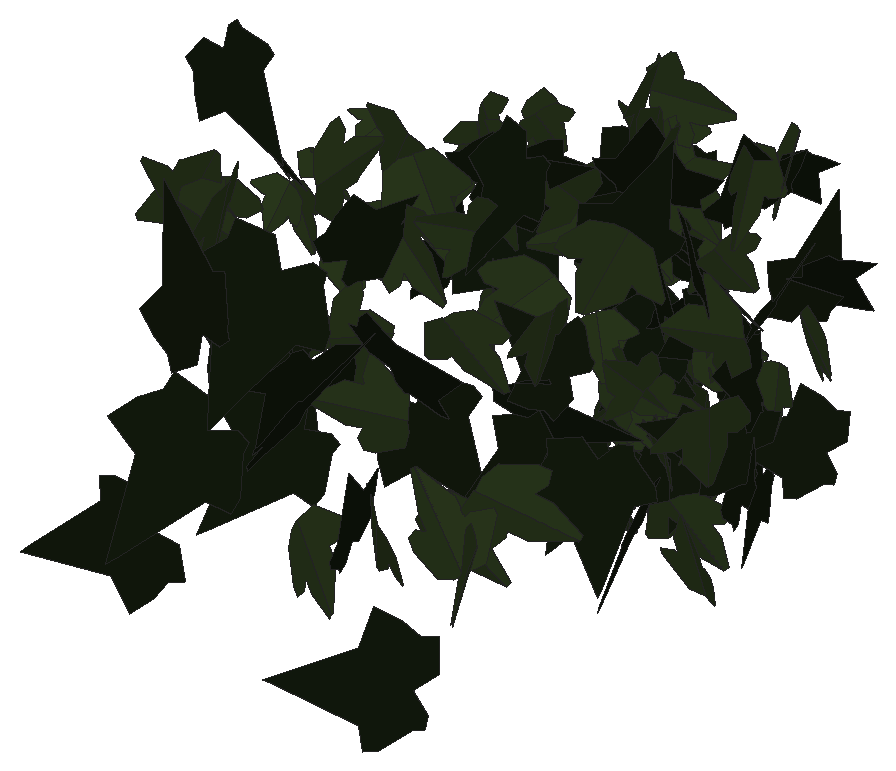
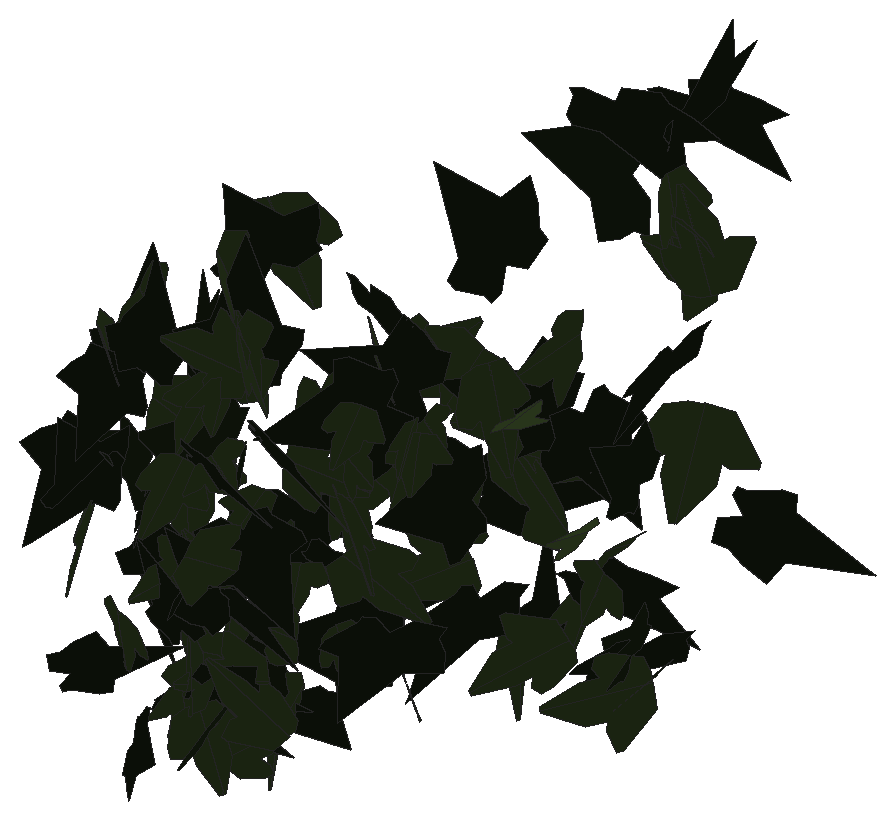
# SketchUp Ruby script. Lengths in inches.
U = 1.inch
M = Sketchup.active_model
def pt(a) = Geom::Point3d.new(a.map { |v| v * U })
def face(e, loops, mat)
  f = e.add_face(loops[0].map { |a| pt(a) })
  loops[1..].each { |l| e.add_face(l.map { |a| pt(a) }).erase! }
  f.material = f.back_material = mat if mat
  f
end
# faces: each face lists its corners as indices into pts; further lists are holes
def faces(e, pts, list, mat = nil) = list.each { |f| face(e, (f[0].is_a?(Array) ? f : [f]).map { |l| l.map { |i| pts[i] } }, mat) }
# xy, xz, yz: faces in a plane at the given z, y or x. An outline is a flat list of corners, or four numbers for a rectangle; further outlines are holes
def ring(l) = l.size == 4 ? [[l[0], l[1]], [l[2], l[1]], [l[2], l[3]], [l[0], l[3]]] : l.each_slice(2).to_a
def flat(e, list, mat, &to3) = list.each { |f| face(e, (f[0].is_a?(Array) ? f : [f]).map { |l| ring(l).map { |u, v| to3.(u, v) } }, mat) }
def xy(e, z, list, mat = nil) = flat(e, list, mat) { |x, y| [x, y, z] }
def xz(e, y, list, mat = nil) = flat(e, list, mat) { |x, z| [x, y, z] }
def yz(e, x, list, mat = nil) = flat(e, list, mat) { |y, z| [x, y, z] }
def lines(e, pts, list) = list.each { |a, b| e.add_line(pt(pts[a]), pt(pts[b])) }
# prism: a flat outline (further loops are holes) pulled along v
def prism(e, loops, v, mat = nil)
  f = face(e, loops, mat); d = Geom::Vector3d.new(v.map { |x| x * U })
  f.pushpull(f.normal.samedirection?(d) ? d.length : -d.length)
end
def box(e, o, s, mat = nil) = prism(e, [[o, [o[0] + s[0], o[1], o[2]], [o[0] + s[0], o[1] + s[1], o[2]], [o[0], o[1] + s[1], o[2]]]], [0, 0, s[2]], mat)
def at(x, y, z, deg = 0) = Geom::Transformation.translation(pt([x, y, z])) * Geom::Transformation.rotation(ORIGIN, Z_AXIS, deg.degrees)
def axes(o, x, y, z) = Geom::Transformation.new([*x, 0, *y, 0, *z, 0, *pt(o).to_a, 1])
def part(name) = M.definitions.add(name)
# library, detail: a bought-in or finely detailed component or shape, given as its bounding box
def library(name, o, s) = part(name).tap { |d| box(d.entities, o, s) }
def detail(e, o, s) = box(e.add_group.entities, o, s)
def put(e, d, t, mat = nil) = e.add_instance(d, t).tap { |i| i.material = mat if mat }
def group(e, t, mat = nil) = e.add_group.tap { |g| g.transformation = t; g.material = mat if mat }.entities
root = M.entities
M.materials.add("efeu1").color = [18, 25, 13]
M.materials.add("efeu2").color = [43, 57, 29]
c1 = part("ivyleaf_9")
p = [[1.54,2.16,1.25],[1.36,2.04,1.19],[-0.21,0.99,0.68],[-0.71,1.11,0.82],[-0.85,0.86,0.67],[-0.8,0.17,0.21],
  [-0.9,-0.01,0.1],[-0.67,-0.16,-0.02],[-0.08,-0.08,-0.05],[-0.03,-0.6,-0.4],[0.65,-0.88,-0.66],[0.83,-0.6,-0.49],
  [1.29,-0.42,-0.43],[1.8125,-0.07,-0.26],[1.21,0.44,0.15]]
faces(c1.entities,p,[[0,1,2,3,4,5,6,7,8,9,10,11,12,13,14]],"efeu1")
c2 = part("ivyleaf_10")
p = [[0,0.5,-0.03],[-0.0625,2.02,-0.43],[-0.19,2.01,-0.46],[-0.54,1.05,-0.29],[-0.52,0.625,-0.18],[-0.83,0.76,-0.28],
  [-1.16,0.64,-0.33],[-1.15,0.33,-0.24],[-0.77,-0.39,0.02],[-0.3,-0.51,0.16],[0.04,-0.48,0.23],[-0.02,2.01,-0.4375],
  [-0.06,2.01,-0.43],[0.04,-0.49,0.23],[0.67,-0.49,0.14],[1.38,0.36,-0.2],[1.375,0.51,-0.24],[0.81,0.65,-0.19],
  [0.62,0.59,-0.15],[0.6,1.09,-0.28],[0.5,1.23,-0.31]]
faces(c2.entities,p,[[0,1,2,3,4,5,6,7,8,9,10],[11,12,0,13,14,15,16,17,18,19,20]],"efeu2")
put(root,c1,axes([595.76,113.43,182.17],[-1.21885,-0.57457,-0.02828],[0.02458,0.01418,-1.34748],[0.57475,-1.21909,-0.00234]))
put(root,c1,axes([593.79,115.78,183.45],[-0.3348,-0.99324,0.75452],[0.23293,0.7177,1.04812],[-1.22538,0.40779,-0.00691]))
put(root,c1,axes([595.95,115.83,181.03],[-0.25255,1.18465,-0.34746],[-0.07372,0.33955,1.21127],[1.23235,0.26308,0.00126]))
put(root,c1,axes([594.6,117.8125,184.29],[-1.21807,-0.67855,-0.32666],[0.28501,0.1596,-1.39432],[0.69707,-1.25097,-0.0007]))
put(root,c1,axes([589.68,118.9,174.91],[-0.19886,-0.25527,-1.12314],[-0.75836,-0.82881,0.32265],[-0.86688,0.78362,-0.02461]))
put(root,c1,axes([597.45,119.31,173.05],[-0.61109,-0.13299,1.02767],[-1.00963,-0.19223,-0.62524],[0.23333,-1.18008,-0.01397]))
put(root,c2,axes([590.875,120.31,184.11],[0.25934,-1.13684,-0.16233],[-0.03169,0.15927,-1.16603],[1.14793,0.26123,0.00448]))
put(root,c1,axes([595.83,120.83,180.86],[0.12584,-0.46219,1.0981],[0.88191,-0.70629,-0.39834],[0.80105,0.85019,0.26604]))
put(root,c2,axes([589.49,121.04,182.95],[-0.11097,0.05172,-1.06693],[0.97659,-0.42966,-0.1224],[-0.43275,-0.98287,-0.00263]))
put(root,c2,axes([589.16,121.18,183.01],[-0.95963,-0.24048,0.45997],[0.45863,0.05985,0.98812],[-0.24303,1.06249,0.04845]))
put(root,c2,axes([596.99,122.26,175.17],[0.59287,-0.92555,-0.33551],[-0.15434,0.29943,-1.09874],[0.97231,0.61188,0.03017]))
put(root,c1,axes([591.73,122.73,178.67],[-0.11706,0.80796,-0.71281],[0.05807,-0.71123,-0.81571],[-1.07588,-0.1263,0.03353]))
put(root,c2,axes([591.73,122.57,173.79],[-0.1766,1.04772,0.235],[-0.04885,0.23007,-1.06245],[-1.07264,-0.18298,0.0097]))
put(root,c2,axes([595.98,123.04,174.75],[0.89607,0.17668,0.6425],[-0.62973,-0.12747,0.91332],[0.21785,-1.09521,-0.00266]))
put(root,c2,axes([593.49,123.5625,177.49],[0.00721,0.0139,1.08365],[-0.97827,-0.46623,0.01249],[0.46635,-0.97825,0.00945]))
put(root,c1,axes([590.07,124.3125,175.47],[-1.12799,-0.42561,0.12182],[-0.11361,-0.04398,-1.20561],[0.42787,-1.13369,0.00104]))
put(root,c1,axes([591.78,124.27,173.13],[0.07336,0.56182,0.80762],[-0.24575,-0.77373,0.56056],[0.95263,-0.24286,0.08241]))
put(root,c2,axes([596.77,123.69,176.26],[-0.50886,-0.25564,-0.97306],[0.91295,0.34087,-0.56698],[0.42275,-1.04384,0.05315]))
put(root,c2,axes([594.42,124.57,174.43],[-0.65237,0.11669,-0.86899],[0.85639,-0.1475,-0.66272],[-0.18804,-1.07656,-0.00339]))
put(root,c2,axes([586.83,124.47,180.89],[-1.00009,-0.64818,-0.21116],[0.17841,0.11296,-1.19177],[0.65795,-1.01588,0.0022]))
put(root,c2,axes([592.375,124.66,173.33],[-0.72851,0.38914,0.66141],[-0.58878,0.30146,-0.82588],[-0.49217,-0.93665,0.00898]))
put(root,c2,axes([590.48,125.66,177.74],[0.44733,-0.25946,-1.05188],[0.88763,-0.56473,0.51678],[-0.62119,-0.99379,-0.01904]))
put(root,c2,axes([598.91,125.7,183.1],[1.03138,0.31187,-0.47094],[-0.5382,0.24508,-1.0164],[-0.17141,1.10701,0.35769]))
put(root,c1,axes([590.9,125.34,180.27],[0.10731,0.01435,1.07001],[0.8971,0.58507,-0.09782],[-0.5834,0.9023,0.0464]))
put(root,c2,axes([590.27,125.17,182.37],[0.0545,-0.04255,-1.07115],[0.22194,1.04975,-0.03041],[1.04877,-0.21994,0.0621]))
put(root,c2,axes([593.74,126.8,181.26],[-0.26991,-0.27088,-0.86435],[-0.5321,-0.68247,0.38004],[-0.73303,0.59514,0.0424]))
put(root,c1,axes([586.27,126.2,183.92],[0.43302,-0.83333,-0.55624],[-0.20808,0.51796,-0.93796],[0.98007,0.47815,0.04663]))
put(root,c2,axes([591.39,126.51,180.49],[0.4739,-0.01093,0.96241],[0.96244,-0.00328,-0.47396],[0.00777,1.07276,0.00836]))
put(root,c1,axes([597.42,126.8125,176.04],[-0.60215,-0.74922,-0.55206],[0.37341,0.40778,-0.96071],[0.85244,-0.70786,0.03088]))
put(root,c2,axes([593.29,126.49,178.5],[-0.84131,-0.15711,-0.51685],[0.50708,0.10011,-0.85584],[0.18624,-0.9823,-0.00456]))
put(root,c2,axes([591.8,126.82,182.12],[0.91415,0.19985,0.59739],[0.57102,0.18164,-0.93457],[-0.26598,1.07682,0.04678]))
put(root,c1,axes([598.48,126.57,182.47],[-0.47235,-0.31422,0.86097],[0.78081,0.36923,0.56313],[-0.47993,0.90997,0.0688]))
put(root,c1,axes([586.63,127.04,175.9],[0.14451,-0.96031,-0.60822],[0.18021,0.62472,-0.94353],[1.12234,0.02334,0.22982]))
put(root,c1,axes([594.51,127.52,183.19],[-1.02084,-0.01927,-0.37602],[0.37509,0.04233,-1.02049],[0.0327,-1.08707,-0.03307]))
put(root,c1,axes([586.19,127.65,181],[0.3789,-0.46509,0.63182],[0.41512,-0.47652,-0.59973],[0.66572,0.56186,0.01436]))
put(root,c1,axes([586.3,127.84,175.02],[-0.03525,-0.76395,0.29627],[0.1508,-0.29753,-0.74924],[0.80539,0.02228,0.15326]))
put(root,c1,axes([591.625,127.09,175.48],[0.19907,-0.73711,-0.86496],[-0.13184,0.85722,-0.76085],[1.12876,0.23012,0.06368]))
put(root,c1,axes([586.11,128.01,176.33],[0.32738,-0.56158,0.45458],[0.22678,-0.39398,-0.65004],[0.686,0.39825,-0.00205]))
put(root,c1,axes([594.34,128.44,174.39],[-0.40105,-0.5135,0.6804],[-0.35041,-0.58616,-0.64892],[0.77708,-0.52934,0.05854]))
put(root,c2,axes([586.49,128.22,179.2],[-0.38884,-0.26504,0.43946],[0.27591,-0.57286,-0.10136],[0.43272,0.1271,0.45953]))
put(root,c2,axes([593.45,128.28,181.31],[0.39931,-0.50089,-0.65183],[0.44093,-0.4811,0.6398],[-0.6938,-0.59403,0.03146]))
put(root,c2,axes([590.63,127.86,182.23],[-0.92116,0.04978,0.59176],[-0.59071,0.03547,-0.9225],[-0.06105,-1.09429,-0.00298]))
put(root,c2,axes([589.29,128.66,181.96],[-0.60664,-0.03869,0.23024],[0.10222,-0.62032,0.16511],[0.2099,0.1903,0.58501]))
put(root,c2,axes([586.2,127.88,175.28],[-0.10763,-0.11667,-1.10556],[0.82861,0.73207,-0.15792],[0.74114,-0.83542,0.01601]))
put(root,c2,axes([594.38,128.67,178.15],[0.01642,-0.94734,0.01205],[0.01069,-0.01187,-0.94742],[0.94736,0.01655,0.01048]))
put(root,c1,axes([592.63,128.31,181.67],[0.35538,-0.03163,0.93868],[0.9392,0.01745,-0.35499],[-0.00513,1.00355,0.03575]))
put(root,c1,axes([598.53,129.28,181],[0.03659,-0.25986,0.90874],[0.18592,-0.88967,-0.26189],[0.9267,0.18875,0.01667]))
put(root,c2,axes([599.45,128.63,177.21],[-0.43752,-0.99419,-0.09924],[0.01792,0.10052,-1.08594],[0.99897,-0.43723,-0.02399]))
put(root,c2,axes([599.05,128.71,172.52],[-0.90111,0.31606,-0.08277],[-0.07933,0.02391,0.95492],[0.31695,0.90459,0.00368]))
put(root,c1,axes([596.99,129.13,173.69],[-0.54469,0.44355,-0.68773],[0.5348,-0.4324,-0.70244],[-0.61944,-0.76334,-0.00171]))
put(root,c1,axes([591.19,128,178.91],[0.25032,0.37607,1.00371],[0.53352,0.85024,-0.45163],[-0.92963,0.58922,0.01108]))
put(root,c2,axes([586.81,129.0625,179.89],[0.01606,-0.6139,0.17619],[0.60651,-0.04057,-0.19666],[0.20015,0.1722,0.58177]))
put(root,c2,axes([586.25,128.93,178.72],[0.65663,-0.08799,0.31882],[0.33056,0.15069,-0.6392],[0.01116,0.71422,0.17414]))
put(root,c2,axes([591.48,129.25,181.48],[0.14816,0.5304,-0.34033],[-0.10692,-0.32338,-0.55054],[-0.62106,0.18221,0.01359]))
put(root,c2,axes([597.52,129.47,183.85],[0.48651,-0.86769,0.40606],[0.19707,-0.35504,-0.99477],[0.93751,0.5249,-0.00161]))
put(root,c1,axes([594.4,129.36,176.42],[-0.76081,-0.26147,-0.45926],[-0.42543,-0.17457,0.80415],[-0.31353,0.87137,0.02329]))
put(root,c2,axes([594.2,130,180.99],[-0.27588,-0.54853,-0.61969],[-0.27584,-0.55492,0.61399],[-0.78026,0.39012,0.00205]))
put(root,c2,axes([599.375,129.5625,179.17],[-0.24554,-0.01347,1.07701],[-1.05783,-0.20495,-0.24373],[0.20278,-1.08547,0.03266]))
put(root,c1,axes([592.9375,129.43,174.72],[0.67331,-0.03723,0.82201],[0.81999,-0.05809,-0.67429],[0.06852,1.06098,-0.00808]))
put(root,c2,axes([595.82,130.39,176.1],[-0.19724,-0.50986,-0.58039],[-0.2319,-0.53231,0.54643],[-0.73691,0.30398,-0.01661]))
put(root,c1,axes([592.9,129.23,181.43],[0.12391,0.43926,-1.00569],[0.24841,0.97459,0.45628],[1.06895,-0.2774,0.01055]))
put(root,c1,axes([596.3,130.33,181.92],[1.02149,0.12938,0.36273],[-0.36153,-0.03213,1.02957],[0.13269,-1.0835,0.01278]))
put(root,c1,axes([598.98,130.65,175.32],[-0.21363,-0.06395,0.97431],[-0.88518,-0.40825,-0.22088],[0.4121,-0.91008,0.03062]))
put(root,c2,axes([594.42,130.46,179.74],[-0.15894,-0.07915,0.84036],[-0.6825,-0.4911,-0.17534],[0.49665,-0.70021,0.02798]))
put(root,c2,axes([596.73,130.29,174.34],[-0.6936,0.443,0.20831],[0.17493,-0.11311,0.823],[0.45721,0.71532,0.00113]))
put(root,c2,axes([592.53,130.48,177.66],[0.75557,0.18129,-0.74961],[-0.72451,-0.19283,-0.77691],[-0.26434,1.04672,-0.01329]))
put(root,c1,axes([598.89,131.12,177.07],[-0.11612,-0.09459,0.97914],[-0.17364,-0.96848,-0.11415],[0.96825,-0.18502,0.09695]))
put(root,c2,axes([590.875,130.38,181.57],[-0.51031,-0.3846,-0.05227],[0.06063,0.0063,-0.63824],[0.38337,-0.51294,0.03136]))
put(root,c1,axes([594.25,131.05,173.38],[-0.662,-0.7157,0.0618],[-0.04417,-0.04332,-0.97491],[0.717,-0.66347,-0.003]))
put(root,c2,axes([592.4375,130.9,180.74],[0.07409,-0.48887,0.43207],[0.18765,-0.4005,-0.48533],[0.62487,0.17824,0.09452]))
put(root,c2,axes([599.04,130.96,183.19],[0.0003,0.88393,-0.54042],[-0.09973,-0.53789,-0.87984],[-1.03124,0.05227,0.08493]))
put(root,c2,axes([591,130.53,182.01],[-0.1537,0.60033,0.17688],[-0.09894,0.15654,-0.61726],[-0.61798,-0.17437,0.05483]))
put(root,c2,axes([597.07,130.54,172.96],[-0.81014,-0.24989,-0.44222],[0.4146,0.15561,-0.84748],[0.29344,-0.90977,-0.02349]))
put(root,c2,axes([592.89,130.87,175.6875],[-0.22211,-0.58425,0.12074],[-0.04729,-0.11119,-0.62503],[0.59472,-0.22704,-0.0046]))
put(root,c2,axes([586.96,130.15,177.15],[0.23523,0.44206,0.95037],[0.46786,0.82731,-0.50062],[-0.93793,0.52355,-0.01137]))
put(root,c1,axes([596.26,130.52,179.3],[0.38903,-0.16104,-0.7006],[-0.64556,0.27222,-0.42104],[0.31628,0.75371,0.00237]))
put(root,c2,axes([594.24,130.8,177.04],[0.41873,0.55255,0.08429],[0.04848,0.06902,-0.69328],[-0.55684,0.42151,0.00303]))
put(root,c1,axes([596.68,131.12,179.8],[0.61048,-0.69246,0.52491],[0.52194,-0.22066,-0.89812],[0.69471,0.77429,0.21349]))
put(root,c1,axes([598.96,130.48,174.01],[-0.07463,0.19995,0.88238],[-0.32805,0.81915,-0.21337],[-0.84318,-0.3364,0.00492]))
put(root,c2,axes([594.41,131.13,175.41],[0.02113,-0.07274,0.90666],[0.90154,0.12189,-0.01123],[-0.12056,0.89867,0.07491]))
put(root,c2,axes([594.89,130.85,172.7],[-0.58796,0.45142,0.38745],[-0.31188,0.22997,-0.74123],[-0.50658,-0.66552,0.00666]))
put(root,c2,axes([592.33,130.99,182.11],[-0.38311,-0.45924,-0.2882],[0.17356,0.23044,-0.59792],[0.51365,-0.42039,-0.01292]))
put(root,c1,axes([598.45,131.55,181.7],[0.52347,0.52675,0.70252],[-0.47395,-0.51901,0.74231],[0.73917,-0.70583,-0.02155]))
put(root,c2,axes([595.3125,131.47,182.24],[-0.7656,0.14191,0.40034],[0.39319,-0.07534,0.77863],[0.16066,0.86066,0.00215]))
put(root,c2,axes([589.97,131.875,176.08],[0.37498,-0.24571,0.89672],[0.74424,-0.50024,-0.44829],[0.55731,0.83336,-0.00469]))
put(root,c1,axes([598.89,131.04,178.47],[-0.35009,0.82077,-0.14824],[-0.05998,0.13558,0.89231],[0.83189,0.35518,0.00195]))
put(root,c1,axes([594.57,131.75,181.04],[-0.95828,0.35686,0.14479],[-0.12979,0.06631,-1.02244],[-0.36259,-0.96689,-0.01668]))
put(root,c2,axes([594.93,131.96,183.72],[0.4008,-0.92985,0.14758],[0.05904,-0.13526,-1.01255],[0.93964,0.40513,0.00068]))
put(root,c2,axes([596.61,131.35,181.58],[0.16398,0.79246,0.40546],[0.04216,0.40491,-0.80842],[-0.88916,0.16535,0.03645]))
put(root,c1,axes([596.4375,132.47,173.81],[-0.37804,-0.81439,0.26484],[0.03259,-0.30297,-0.88512],[0.85575,-0.34823,0.15071]))
put(root,c2,axes([593.82,131.43,174.03],[-0.04222,0.10841,0.65697],[-0.34329,0.56052,-0.11455],[-0.57054,-0.34528,0.02031]))
put(root,c1,axes([595.83,131.93,173.04],[-0.37373,-0.15928,-0.74864],[-0.70331,-0.25723,0.40582],[-0.30198,0.79622,-0.01865]))
put(root,c2,axes([595.98,132.04,176.35],[-0.64507,-0.01848,0.55003],[0.55004,0.00643,0.6453],[-0.01823,0.84771,0.0071]))
put(root,c2,axes([594.85,131.71,179.24],[0.14668,0.57488,0.38881],[0.0805,0.38062,-0.59315],[-0.68933,0.16678,0.01347]))
put(root,c1,axes([596.13,132.78,176.9375],[0.2465,-0.47253,-0.63524],[0.38033,-0.51285,0.52907],[-0.69438,-0.44864,0.06428]))
put(root,c1,axes([595.1875,132.45,176.69],[-0.95624,-0.08571,-0.10025],[0.10141,-0.00865,-0.95991],[0.08433,-0.96144,0.01757]))
put(root,c2,axes([595.58,132.43,180.4],[0.22932,0.64542,-0.37861],[-0.11528,-0.36079,-0.68486],[-0.73933,0.25645,-0.01064]))
put(root,c2,axes([595.57,132.09,182.35],[0.14522,0.72702,0.08078],[0.01261,0.07986,-0.74137],[-0.73138,0.14573,0.00326]))
put(root,c2,axes([595.67,132.53,173.21],[-0.057,0.04209,0.78568],[-0.67663,-0.40464,-0.02741],[0.40154,-0.67588,0.06534]))
put(root,c2,axes([596.42,132.38,173.67],[0.25943,0.7715,-0.15752],[-0.06129,-0.14556,-0.81387],[-0.78503,0.26633,0.01149]))
put(root,c2,axes([594.83,132.59,172.46],[0.35847,0.3433,0.59824],[-0.46096,-0.3823,0.49559],[0.51309,-0.58331,0.02728]))
put(root,c2,axes([595.16,132.3125,183.16],[-0.11086,-0.02441,1.00018],[0.95837,0.28626,0.11321],[-0.28717,0.96473,-0.00829]))
put(root,c2,axes([594.73,132.08,174.4],[0.13707,0.03484,0.93038],[0.72417,0.58705,-0.12867],[-0.58514,0.73469,0.0587]))
put(root,c2,axes([597,132.1875,179.41],[-0.37352,-0.60882,-0.48516],[0.25443,0.4131,-0.71427],[0.73574,-0.45194,0.0007]))
put(root,c2,axes([596.88,131.9,176.74],[0.11269,0.18418,0.78639],[0.13453,0.77864,-0.20165],[-0.79639,0.15759,0.07722]))
put(root,c2,axes([598.77,132.71,182.82],[0.59366,-0.73168,0.1017],[0.06415,-0.07892,-0.94223],[0.73593,0.59711,0.00009]))
put(root,c1,axes([595.29,132.98,174.39],[-0.71167,-0.22359,0.5145],[-0.48878,-0.16072,-0.74595],[0.27531,-0.86334,0.00562]))
put(root,c1,axes([594.5,132.6,178.79],[0.25367,0.55947,-0.77825],[-0.31641,-0.71103,-0.61429],[-0.90475,0.40553,-0.00338]))
put(root,c1,axes([590.04,132.54,177.49],[-0.20473,-0.75246,-0.7988],[0.21747,0.76864,-0.7798],[1.07563,-0.29862,0.00562]))
put(root,c1,axes([596.45,132.72,175.62],[-0.24439,0.1777,0.76249],[0.53451,-0.54578,0.29851],[0.57206,0.58587,0.04682]))
put(root,c1,axes([595.15,132.58,176.77],[0.38993,0.6786,0.01311],[-0.00955,-0.00964,0.78264],[0.67866,-0.39003,0.00347]))
put(root,c2,axes([591.09,132.86,180.75],[0.82059,-0.62751,-0.26292],[-0.21013,0.15804,-1.03302],[0.6471,0.84707,-0.00204]))
put(root,c1,axes([595.78,132.84,180.5],[-0.70639,0.32195,0.32528],[-0.29993,0.12622,-0.77625],[-0.34569,-0.76737,0.00879]))
put(root,c2,axes([595.6,133.16,174.1],[-0.62567,0.19975,0.5243],[0.46689,-0.25013,0.65246],[0.31113,0.77704,0.07525]))
put(root,c1,axes([594.78,133.61,173.68],[0.22341,-0.82251,0.41936],[0.11805,-0.40247,-0.85228],[0.91567,0.25257,0.00756]))
put(root,c2,axes([595.43,133.16,173.42],[-0.76339,-0.24462,0.40341],[-0.38442,-0.12232,-0.80162],[0.2735,-0.85471,-0.00073]))
put(root,c1,axes([599.19,132.86,178.64],[-0.31906,-0.44734,0.78963],[0.58921,0.5345,0.54089],[-0.69025,0.66304,0.09671]))
put(root,c2,axes([595.03,133.67,178.4],[0.27012,0.36267,-0.81961],[-0.58303,-0.57904,-0.44837],[-0.68071,0.63987,0.05879]))
put(root,c1,axes([597.08,133.67,172.49],[-0.09707,0.09646,-0.77419],[0.63858,-0.43838,-0.13469],[-0.44821,-0.64546,-0.02422]))
put(root,c2,axes([597.66,133.42,175.61],[0.7395,-0.2878,0.21417],[0.20363,-0.06723,-0.79346],[0.29535,0.76695,0.01082]))
put(root,c1,axes([598.9,133.74,173.9],[-0.4392,-0.01102,0.83666],[-0.77668,-0.34614,-0.41227],[0.31126,-0.87925,0.15182]))
put(root,c1,axes([599.27,132.68,179.38],[0.64688,0.68241,0.17418],[0.11404,0.13188,-0.94025],[-0.69499,0.65681,0.00783]))
put(root,c1,axes([598.28,132.93,182.08],[0.5244,0.58671,-0.02513],[-0.01683,-0.01866,-0.78691],[-0.58701,0.52467,0.00011]))
put(root,c2,axes([599.17,132.97,177.79],[-0.51662,0.70695,0.40574],[-0.22524,0.33785,-0.87545],[-0.78337,-0.56336,-0.01586]))
put(root,c2,axes([593.17,133.24,174.27],[0.69213,-0.04297,-0.81937],[0.82031,0.01368,0.69221],[-0.01726,-1.07249,0.04165]))
